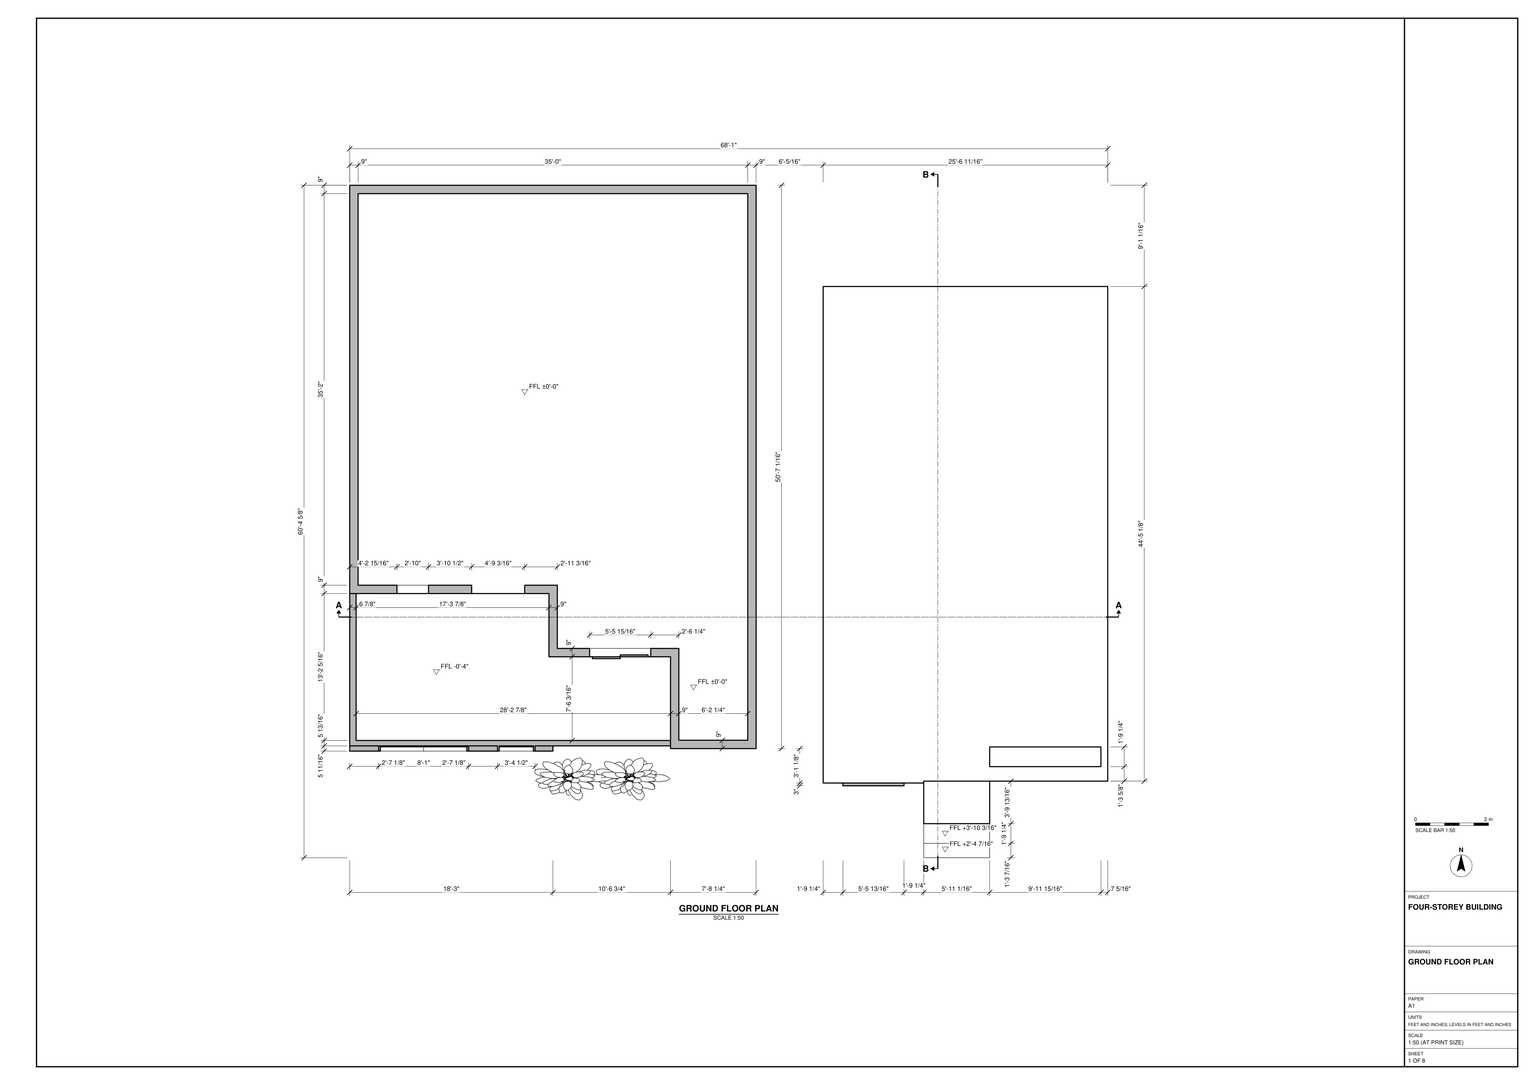
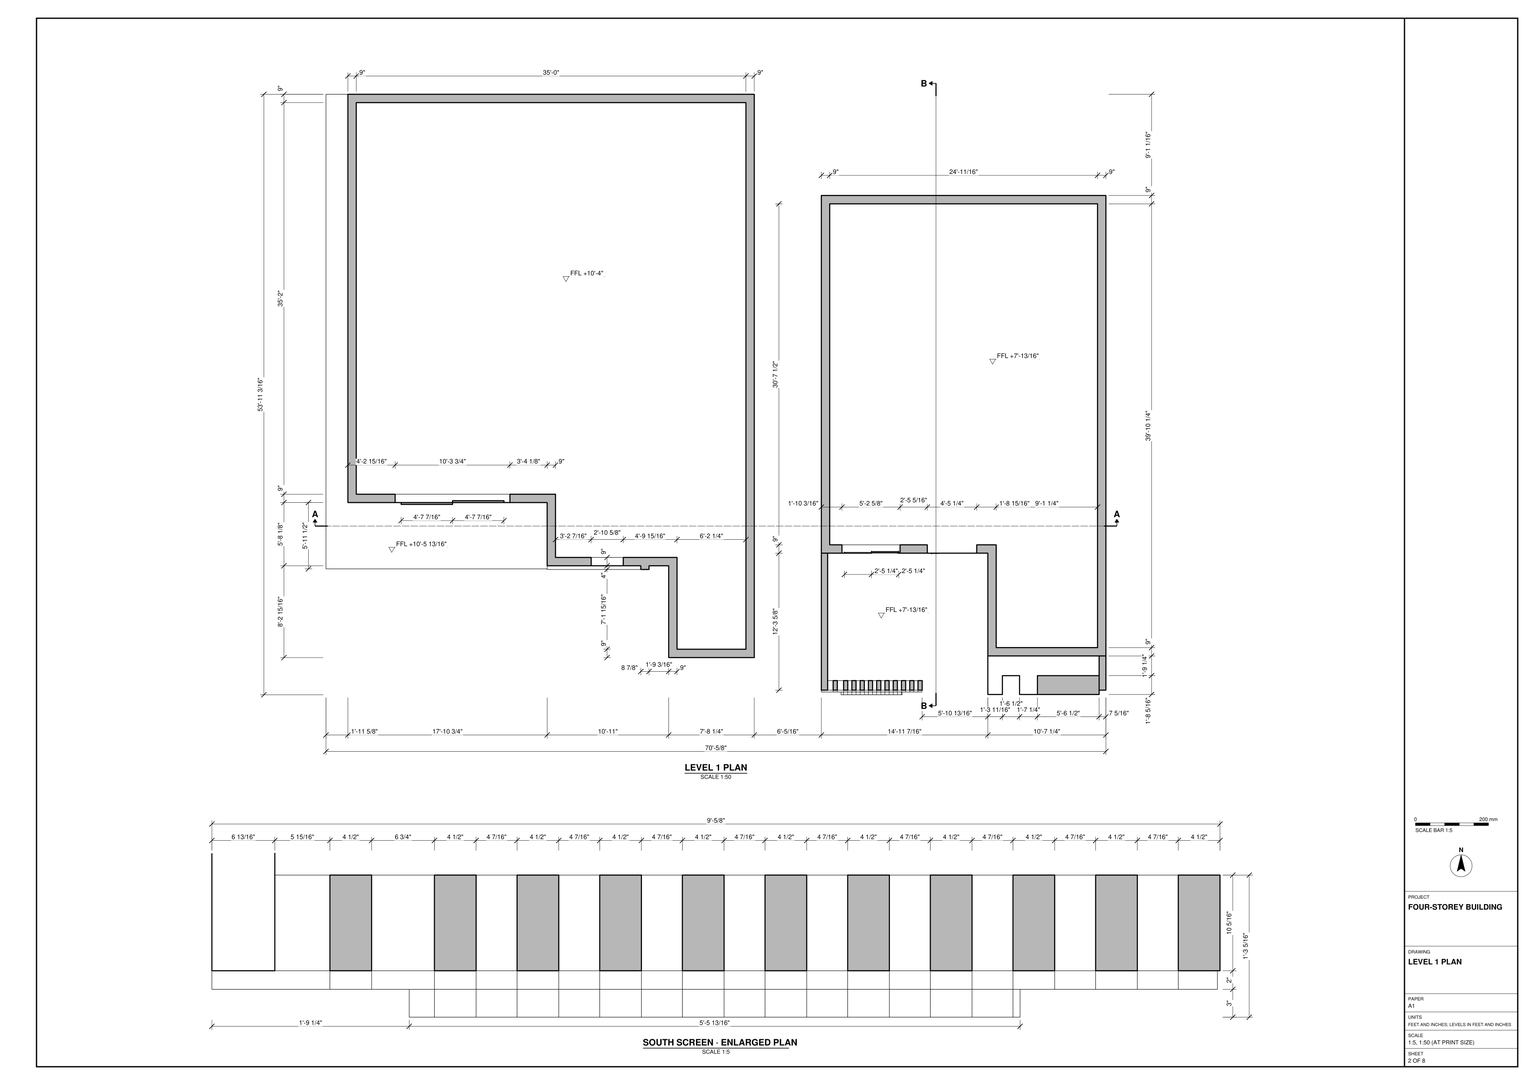
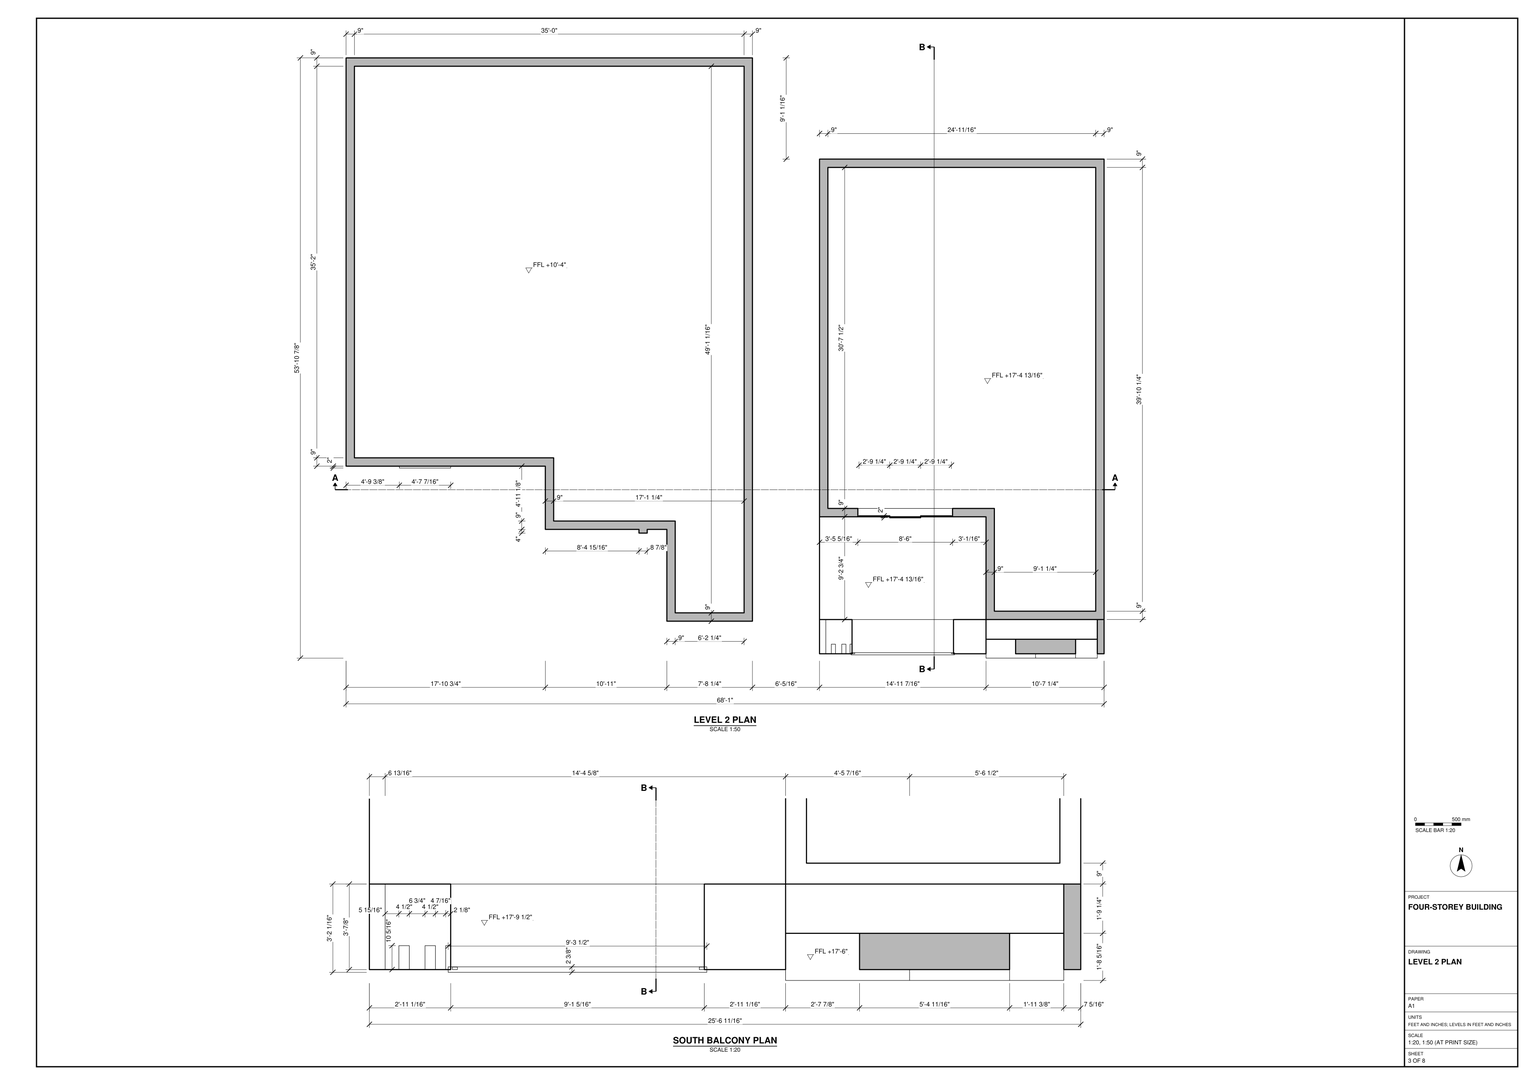
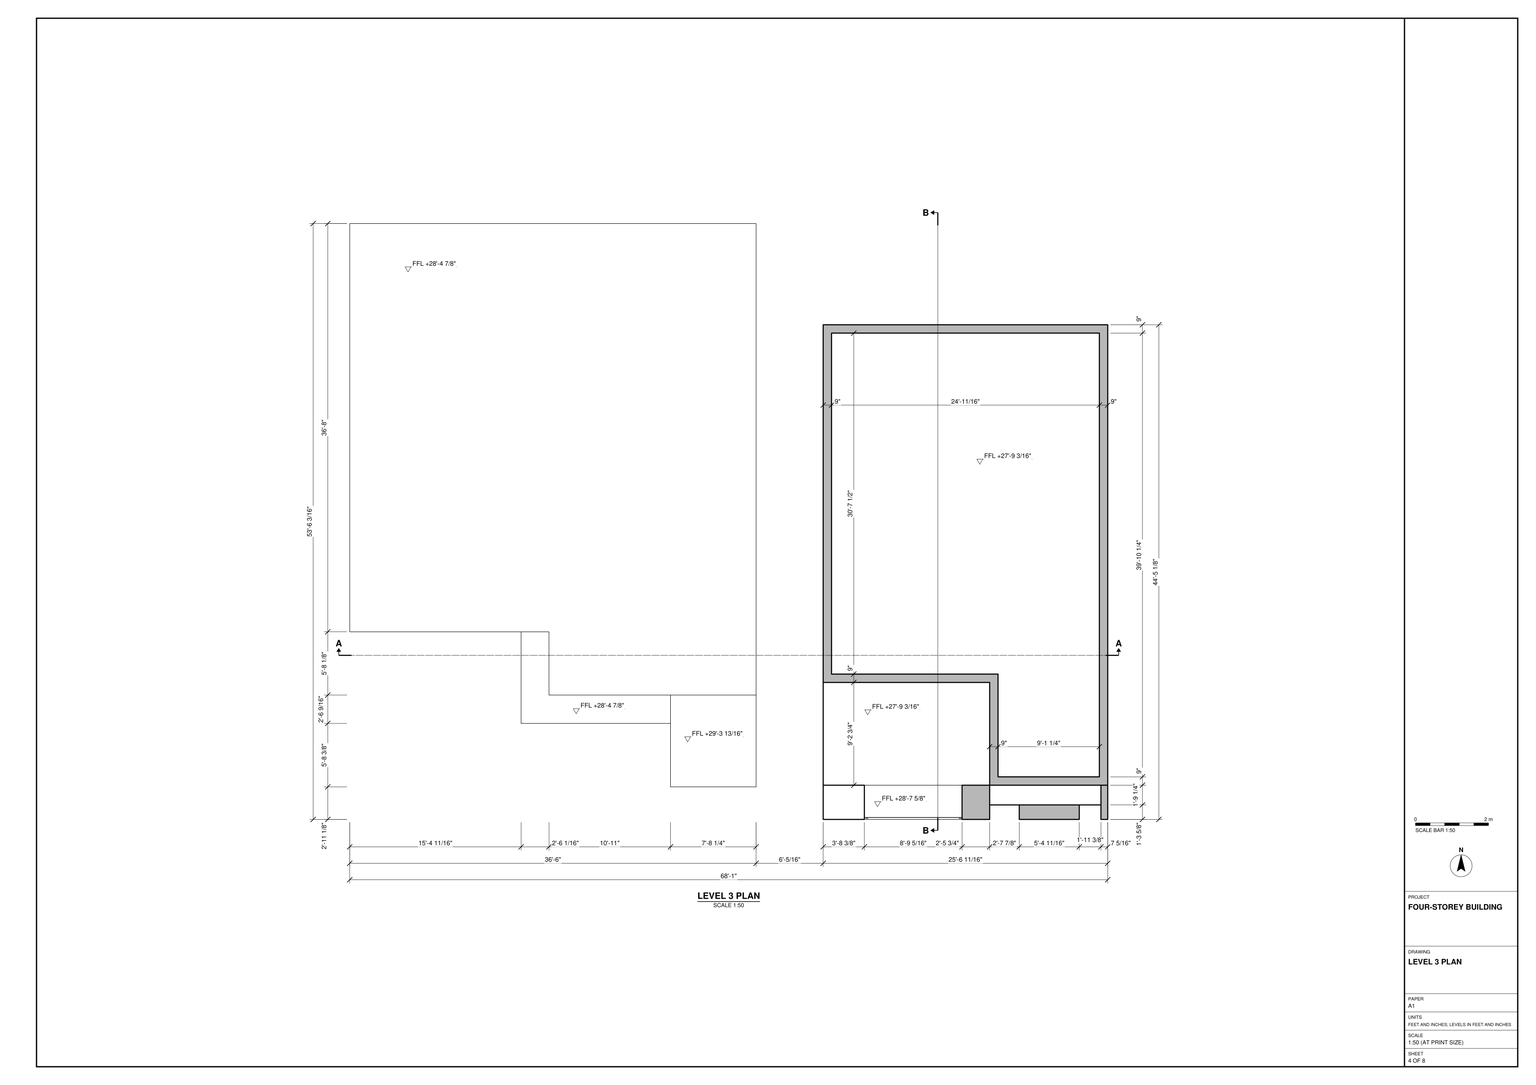
Build the four-storey building in SketchUp from task_files/diagram_01.pdf. Work in feet and inches. The completed model shall measure 70'-5/8" along X, 60'-4 5/8" along Y and 38'-9 3/4" along Z. Use the storey levels ±0'-0", +10'-4", +17'-4 13/16" and +28'-4 7/8" relative to the ground floor. Follow the floor levels marked in each wing rather than extending every slab across both wings.

Place the wider wing to the west and the narrower wing to the east, with the gap and the north–south offset shown in plan. Trace each floor separately to capture the stepped south walls of the west wing and the recessed frontage of the east wing. Model the walls at their drawn thicknesses, including the 9" walls, and place the door and window openings in the corresponding wall segments. Include the floor slabs, entrance steps, roof, and any built-in joinery and main furniture shown. Use the enlarged plans to set out the individual fins of the east wing's south screen and the edges and returns of the balcony above.

Keep walls, slabs, roof elements and individual furniture or joinery pieces in separate groups or components. Use components for repeated parts such as screen fins. Decor and loose items may be any suitable library components. Save one SketchUp model as output_files/four_storey_building_with_offset_wings.skp.

# SketchUp Ruby script. Lengths in inches.
U = 1.inch
M = Sketchup.active_model
def pt(a) = Geom::Point3d.new(a.map { |v| v * U })
def face(e, loops, mat)
  f = e.add_face(loops[0].map { |a| pt(a) })
  loops[1..].each { |l| e.add_face(l.map { |a| pt(a) }).erase! }
  f.material = f.back_material = mat if mat
  f
end
# faces: each face lists its corners as indices into pts; further lists are holes
def faces(e, pts, list, mat = nil) = list.each { |f| face(e, (f[0].is_a?(Array) ? f : [f]).map { |l| l.map { |i| pts[i] } }, mat) }
# xy, xz, yz: faces in a plane at the given z, y or x. An outline is a flat list of corners, or four numbers for a rectangle; further outlines are holes
def ring(l) = l.size == 4 ? [[l[0], l[1]], [l[2], l[1]], [l[2], l[3]], [l[0], l[3]]] : l.each_slice(2).to_a
def flat(e, list, mat, &to3) = list.each { |f| face(e, (f[0].is_a?(Array) ? f : [f]).map { |l| ring(l).map { |u, v| to3.(u, v) } }, mat) }
def xy(e, z, list, mat = nil) = flat(e, list, mat) { |x, y| [x, y, z] }
def xz(e, y, list, mat = nil) = flat(e, list, mat) { |x, z| [x, y, z] }
def yz(e, x, list, mat = nil) = flat(e, list, mat) { |y, z| [x, y, z] }
def lines(e, pts, list) = list.each { |a, b| e.add_line(pt(pts[a]), pt(pts[b])) }
# prism: a flat outline (further loops are holes) pulled along v
def prism(e, loops, v, mat = nil)
  f = face(e, loops, mat); d = Geom::Vector3d.new(v.map { |x| x * U })
  f.pushpull(f.normal.samedirection?(d) ? d.length : -d.length)
end
def box(e, o, s, mat = nil) = prism(e, [[o, [o[0] + s[0], o[1], o[2]], [o[0] + s[0], o[1] + s[1], o[2]], [o[0], o[1] + s[1], o[2]]]], [0, 0, s[2]], mat)
def at(x, y, z, deg = 0) = Geom::Transformation.translation(pt([x, y, z])) * Geom::Transformation.rotation(ORIGIN, Z_AXIS, deg.degrees)
def axes(o, x, y, z) = Geom::Transformation.new([*x, 0, *y, 0, *z, 0, *pt(o).to_a, 1])
def part(name) = M.definitions.add(name)
# library, detail: a bought-in or finely detailed component or shape, given as its bounding box
def library(name, o, s) = part(name).tap { |d| box(d.entities, o, s) }
def detail(e, o, s) = box(e.add_group.entities, o, s)
def put(e, d, t, mat = nil) = e.add_instance(d, t).tap { |i| i.material = mat if mat }
def group(e, t, mat = nil) = e.add_group.tap { |g| g.transformation = t; g.material = mat if mat }.entities
root = M.entities
M.materials.add("Material__1").color = [190, 136, 85]
M.materials.add("Material__2").color = [51, 42, 44]
M.materials.add("Material__3").color = [119, 136, 107]
M.materials.add("[Cladding Weathered]").color = [109, 103, 94]
M.materials.add("[Color C02]").color = [255, 204, 153]
M.materials.add("[Color C07]").color = [153, 76, 0]
M.materials.add("[Color L16]").color = [102, 0, 51]
M.materials.add("[Color M02]").color = [198, 198, 198]
M.materials.add("[Color M03]").color = [170, 170, 170]
M.materials.add("[Color M04]").color = [142, 142, 142]
M.materials.add("[Color M05]").color = [114, 114, 114]
M.materials.add("[Color M06]").color = [86, 86, 86]
M.materials.add("[Color M08]").color = [30, 30, 30]
M.materials.add("[Color M09]").color = [0, 0, 0]
M.materials.add("[Formica Laminate Light]").color = [213, 189, 164]
M.materials.add("[Stone Random Rubble]").color = [91, 91, 91]
M.materials.add("[Stone Vein Gray]").color = [166, 165, 165]
M.materials.add("[Tile Veriegated Stone]").color = [171, 137, 112]
M.materials.add("[Translucent Glass Blue]").color = [7, 17, 153]
M.materials["[Translucent Glass Blue]"].alpha = 0.5
M.materials.add("[Translucent Glass Blue]1").color = [100, 149, 237]
M.materials["[Translucent Glass Blue]1"].alpha = 0.5
M.materials.add("[Translucent Glass Tinted]").color = [8, 201, 241]
M.materials["[Translucent Glass Tinted]"].alpha = 0.48
M.materials.add("[Wood Cherry Original]").color = [152, 86, 42]
c1 = library("\#2",[-119.83,-119.83,113.8],[239.66,239.66,17.4])
c2 = library("\#4",[-204.92,-212.35,-236.71],[424.28,257.5,472.53])
c3 = part("\#3")
put(c3.entities,c2,axes([-0.37,309.72,0],[1.36765,0,0],[0,1.36765,0],[0,0,1.36765]),"Material__3")
c4 = part("Difference\#1")
xy(c4.entities,0,[[345.75,0,345.75,98.9375,324.5625,98.9375,324.5625,94.9375,315.6875,94.9375,315.6875,98.9375,214.75,98.9375,214.75,167.0625,188.59,167.0625,188.59,176.0625,223.75,176.0625,223.75,107.9375,354.75,107.9375,354.75,9,429,9,429,598.0625,9,598.0625,9,176.0625,188.59,176.0625,188.59,167.0625,0,167.0625,0,607.0625,438,607.0625,438,0]])
xy(c4.entities,1.81,[[50.92,167.0625,174.65,176.0625]])
xy(c4.entities,12.375,[[262.1875,98.9375,296.8,107.9375]])
xy(c4.entities,107.98,[[50.92,167.0625,174.65,176.0625]])
xy(c4.entities,124.625,[[262.1875,98.9375,296.8,107.9375]])
xy(c4.entities,138.9,[[0,94.9375,0,167.0625,214.75,167.0625,214.75,98.9375,315.6875,98.9375,315.6875,94.9375]],"[Color M02]")
xy(c4.entities,152.125,[[0,94.9375,324.5625,94.9375,324.5625,98.9375,214.75,98.9375,214.75,167.0625,0,167.0625]],"[Color M08]")
xy(c4.entities,212.875,[[[345.75,0,438,0,438,607.0625,0,607.0625,0,167.0625,214.75,167.0625,214.75,98.9375,345.75,98.9375],[354.75,9,354.75,107.9375,223.75,107.9375,223.75,176.0625,9,176.0625,9,598.0625,429,598.0625,429,9]]])
xz(c4.entities,0,[[345.75,0,438,212.875]])
xz(c4.entities,9,[[354.75,0,429,212.875]])
xz(c4.entities,94.9375,[[315.6875,0,324.5625,0,324.5625,152.125,0,152.125,0,138.9,315.6875,138.9]],"[Color M08]")
xz(c4.entities,98.9375,[[324.5625,0,345.75,0,345.75,212.875,214.75,212.875,214.75,152.125,324.5625,152.125],[[214.75,0,315.6875,138.9],[262.1875,12.375,296.8,124.625]]])
xz(c4.entities,107.9375,[[[223.75,0,354.75,212.875],[262.1875,12.375,296.8,124.625]]])
xz(c4.entities,167.0625,[[[0,0,214.75,138.9],[50.92,1.81,174.65,107.98]],[0,138.9,214.75,152.125],[0,152.125,214.75,212.875]])
xz(c4.entities,176.0625,[[[9,0,223.75,212.875],[50.92,1.81,174.65,107.98]]])
xz(c4.entities,598.0625,[[9,0,429,212.875]])
xz(c4.entities,607.0625,[[0,0,438,212.875]])
yz(c4.entities,0,[[167.0625,0,607.0625,212.875]])
yz(c4.entities,0,[[94.9375,138.9,167.0625,152.125]],"[Color M08]")
yz(c4.entities,9,[[176.0625,0,598.0625,212.875]])
yz(c4.entities,50.92,[[167.0625,1.81,176.0625,107.98]])
yz(c4.entities,174.65,[[167.0625,1.81,176.0625,107.98]])
yz(c4.entities,214.75,[[98.9375,0,167.0625,138.9],[98.9375,152.125,167.0625,212.875]])
yz(c4.entities,223.75,[[107.9375,0,176.0625,212.875]])
yz(c4.entities,262.1875,[[98.9375,12.375,107.9375,124.625]])
yz(c4.entities,296.8,[[98.9375,12.375,107.9375,124.625]])
yz(c4.entities,315.6875,[[94.9375,0,98.9375,138.9]])
yz(c4.entities,324.5625,[[94.9375,0,98.9375,152.125]])
yz(c4.entities,345.75,[[0,0,98.9375,212.875]])
yz(c4.entities,354.75,[[9,0,107.9375,212.875]])
yz(c4.entities,429,[[9,0,598.0625,212.875]])
yz(c4.entities,438,[[0,0,607.0625,212.875]])
c5 = part("Group\#3")
box(c5.entities,[0,-2,0],[55.41,2,93.24])
c6 = library("Slatted screen panel \#1",[0,-1,-56.29],[36.84,1,58.71])
c7 = library("Group\#11",[0,-1,-55.71],[93.48,1,58.6])
c8 = part("Difference\#2")
xy(c8.entities,0,[[345.75,0,345.75,98.9375,214.75,98.9375,214.75,167.0625,188.59,167.0625,188.59,176.0625,223.75,176.0625,223.75,107.9375,354.75,107.9375,354.75,9,429,9,429,598.0625,9,598.0625,9,176.0625,131.41,176.0625,131.41,167.0625,0,167.0625,0,607.0625,438,607.0625,438,0]])
xy(c8.entities,12.41,[[50.92,167.0625,84.9,176.0625]])
xy(c8.entities,42.9375,[[258.5625,98.9375,324.49,107.9375]])
xy(c8.entities,93.0625,[[131.41,167.0625,188.59,176.0625]])
xy(c8.entities,98.98,[[50.92,167.0625,84.9,176.0625]])
xy(c8.entities,109.0625,[[258.5625,98.9375,324.49,107.9375]])
xy(c8.entities,120,[[[345.75,0,438,0,438,607.0625,0,607.0625,0,167.0625,214.75,167.0625,214.75,98.9375,345.75,98.9375],[354.75,9,354.75,107.9375,223.75,107.9375,223.75,176.0625,9,176.0625,9,598.0625,429,598.0625,429,9]]])
xz(c8.entities,0,[[345.75,0,438,120]])
xz(c8.entities,9,[[354.75,0,429,120]])
xz(c8.entities,98.9375,[[[214.75,0,345.75,120],[258.5625,42.9375,324.49,109.0625]]])
xz(c8.entities,98.9375,[[[258.5625,42.9375,324.49,109.0625],[261.47,45.85,321.58,106.15]]],"[Color M09]")
xz(c8.entities,107.9375,[[[223.75,0,354.75,120],[258.5625,42.9375,324.49,109.0625]]])
xz(c8.entities,167.0625,[[[0,0,131.41,0,131.41,93.0625,188.59,93.0625,188.59,0,214.75,0,214.75,120,0,120],[50.92,12.41,84.9,98.98]]])
xz(c8.entities,167.0625,[[[50.92,12.41,84.9,98.98],[53.26,14.76,82.56,96.63]]],"[Color M09]")
xz(c8.entities,167.0625,[[53.26,14.76,82.56,96.63]],"[Translucent Glass Tinted]")
xz(c8.entities,176.0625,[[[9,0,9,120,223.75,120,223.75,0,188.59,0,188.59,93.0625,131.41,93.0625,131.41,0],[50.92,12.41,84.9,98.98]]])
xz(c8.entities,598.0625,[[9,0,429,120]])
xz(c8.entities,607.0625,[[0,0,438,120]])
yz(c8.entities,0,[[167.0625,0,607.0625,120]])
yz(c8.entities,9,[[176.0625,0,598.0625,120]])
yz(c8.entities,50.92,[[167.0625,12.41,176.0625,98.98]])
yz(c8.entities,84.9,[[167.0625,12.41,176.0625,98.98]])
yz(c8.entities,131.41,[[167.0625,0,176.0625,93.0625]])
yz(c8.entities,188.59,[[167.0625,0,176.0625,93.0625]])
yz(c8.entities,214.75,[[98.9375,0,167.0625,120]])
yz(c8.entities,223.75,[[107.9375,0,176.0625,120]])
yz(c8.entities,258.5625,[[98.9375,42.9375,107.9375,109.0625]])
yz(c8.entities,324.49,[[98.9375,42.9375,107.9375,109.0625]])
yz(c8.entities,345.75,[[0,0,98.9375,120]])
yz(c8.entities,354.75,[[9,0,107.9375,120]])
yz(c8.entities,429,[[9,0,598.0625,120]])
yz(c8.entities,438,[[0,0,607.0625,120]])
g1 = group(c8.entities,at(261.47,96.9375,45.85))
g2 = group(g1,at(0,2,0),"[Translucent Glass Tinted]")
box(g2,[0,-2,0],[30.05,2,60.3])
g3 = group(g1,at(30.05,4,0),"[Translucent Glass Tinted]")
box(g3,[0,-2,0],[30.05,2,60.3])
c9 = library("\#1",[-174.07,-174.07,0],[348.14,348.14,140])
c10 = part("Difference\#4")
xy(c10.entities,0,[[179.4375,0,179.4375,110.75,167.47,110.75,167.47,119.75,188.4375,119.75,188.4375,9,297.6875,9,297.6875,487.23,9,487.23,9,119.75,114.1875,119.75,114.1875,110.75,0,110.75,0,496.23,306.6875,496.23,306.6875,0]])
xy(c10.entities,25.61,[[22.2,110.75,84.85,119.75]])
xy(c10.entities,90.42,[[22.2,110.75,84.85,119.75]])
xy(c10.entities,102.6875,[[114.1875,110.75,167.47,119.75]])
xy(c10.entities,120,[[[179.4375,0,306.6875,0,306.6875,496.23,0,496.23,0,110.75,179.4375,110.75],[188.4375,9,188.4375,119.75,9,119.75,9,487.23,297.6875,487.23,297.6875,9]]])
xz(c10.entities,0,[[179.4375,0,306.6875,120]])
xz(c10.entities,9,[[188.4375,0,297.6875,120]])
xz(c10.entities,110.75,[[[0,0,114.1875,0,114.1875,102.6875,167.47,102.6875,167.47,0,179.4375,0,179.4375,120,0,120],[22.2,25.61,84.85,90.42]]])
xz(c10.entities,119.75,[[[9,0,9,120,188.4375,120,188.4375,0,167.47,0,167.47,102.6875,114.1875,102.6875,114.1875,0],[22.2,25.61,84.85,90.42]]])
xz(c10.entities,487.23,[[9,0,297.6875,120]])
xz(c10.entities,496.23,[[0,0,306.6875,120]])
yz(c10.entities,0,[[110.75,0,496.23,120]])
yz(c10.entities,9,[[119.75,0,487.23,120]])
yz(c10.entities,22.2,[[110.75,25.61,119.75,90.42]])
yz(c10.entities,84.85,[[110.75,25.61,119.75,90.42]])
yz(c10.entities,114.1875,[[110.75,0,119.75,102.6875]])
yz(c10.entities,167.47,[[110.75,0,119.75,102.6875]])
yz(c10.entities,179.4375,[[0,0,110.75,120]])
yz(c10.entities,188.4375,[[9,0,119.75,120]])
yz(c10.entities,297.6875,[[9,0,487.23,120]])
yz(c10.entities,306.6875,[[0,0,496.23,120]])
c11 = part("Group\#12")
box(c11.entities,[0,0,0],[306.6875,496.23,4])
c12 = part("Difference")
xy(c12.entities,0,[[[179.4375,0,179.4375,110.75,0,110.75,0,496.23,306.6875,496.23,306.6875,0],[188.4375,9,297.6875,9,297.6875,487.23,9,487.23,9,119.75,188.4375,119.75]]])
xy(c12.entities,25.61,[[41.33,110.75,143.35,119.75]])
xy(c12.entities,90.42,[[41.33,110.75,143.35,119.75]])
xy(c12.entities,120,[[[179.4375,0,306.6875,0,306.6875,496.23,0,496.23,0,110.75,179.4375,110.75],[188.4375,9,188.4375,119.75,9,119.75,9,487.23,297.6875,487.23,297.6875,9]]])
xz(c12.entities,0,[[179.4375,0,306.6875,120]])
xz(c12.entities,9,[[188.4375,0,297.6875,120]])
xz(c12.entities,110.75,[[[0,0,179.4375,120],[41.33,25.61,143.35,90.42]]])
xz(c12.entities,119.75,[[[9,0,188.4375,120],[41.33,25.61,143.35,90.42]]])
xz(c12.entities,487.23,[[9,0,297.6875,120]])
xz(c12.entities,496.23,[[0,0,306.6875,120]])
yz(c12.entities,0,[[110.75,0,496.23,120]])
yz(c12.entities,9,[[119.75,0,487.23,120]])
yz(c12.entities,41.33,[[110.75,25.61,119.75,90.42]])
yz(c12.entities,143.35,[[110.75,25.61,119.75,90.42]])
yz(c12.entities,179.4375,[[0,0,110.75,120]])
yz(c12.entities,188.4375,[[9,0,119.75,120]])
yz(c12.entities,297.6875,[[9,0,487.23,120]])
yz(c12.entities,306.6875,[[0,0,496.23,120]])
c13 = part("Difference\#3")
xy(c13.entities,0,[[179.4375,0,179.4375,110.75,167.47,110.75,167.47,119.75,188.4375,119.75,188.4375,9,297.6875,9,297.6875,487.23,9,487.23,9,119.75,114.1875,119.75,114.1875,110.75,0,110.75,0,496.23,306.6875,496.23,306.6875,0],[114.1875,110.75,167.47,119.75]])
xy(c13.entities,120,[[[179.4375,0,306.6875,0,306.6875,496.23,0,496.23,0,110.75,179.4375,110.75],[188.4375,9,188.4375,119.75,9,119.75,9,487.23,297.6875,487.23,297.6875,9]]])
xz(c13.entities,0,[[179.4375,0,306.6875,120]])
xz(c13.entities,9,[[188.4375,0,297.6875,120]])
xz(c13.entities,110.75,[[0,0,179.4375,120]])
xz(c13.entities,119.75,[[9,0,188.4375,120]])
xz(c13.entities,487.23,[[9,0,297.6875,120]])
xz(c13.entities,496.23,[[0,0,306.6875,120]])
yz(c13.entities,0,[[110.75,0,496.23,120]])
yz(c13.entities,9,[[119.75,0,487.23,120]])
yz(c13.entities,179.4375,[[0,0,110.75,120]])
yz(c13.entities,188.4375,[[9,0,119.75,120]])
yz(c13.entities,297.6875,[[9,0,487.23,120]])
yz(c13.entities,306.6875,[[0,0,496.23,120]])
c14 = part("Group28\#1")
box(c14.entities,[711.27,-0.8125,128.69],[2.16,2.16,33.63])
c15 = part("Group29\#1")
box(c15.entities,[820.61,-0.8125,128.69],[2.17,2.16,33.63])
c16 = part("Group31\#1")
box(c16.entities,[711.27,-0.91,162.32],[111.51,2.36,2.37])
c17 = part("Group32\#1")
box(c17.entities,[712.35,-0.71,132.62],[109.35,1.96,1.97])
c18 = library("Group33\#1",[712.35,0.27,134.59],[109.35,0.01,27.73])
c19 = library("Group\#20",[0,-20.3125,-118.5],[66.48,20.3125,125.22])
xy(root,-4,[[30.5,126.31,369.375,126.31,369.375,216.52,238.375,216.52,238.375,284.65,30.5,284.65]])
xy(root,3.92,[[[533.92,80.48,533.92,615.59,840.61,615.59,840.61,82.48,642.3,82.48,642.3,80.48],[713.36,98.11,833.29,119.36]]])
xy(root,28.42,[[642.3,0,713.36,15.42]])
xy(root,46.17,[[642.3,15.42,713.36,36.67]])
xy(root,64.17,[[642.3,36.67,713.36,56.48]])
xy(root,73.4,[[713.36,77.79,840.61,82.48]])
xy(root,84.8,[[642.3,56.48,713.36,82.48],[766.81,77.79,840.61,77.79,840.61,615.59,533.92,615.59,533.92,80.48,642.3,80.48,642.3,82.48,713.36,82.48,713.36,119.36,833.29,119.36,833.29,98.11,766.81,98.11],[713.36,77.79,766.81,98.11],[713.36,98.11,833.29,119.36]])
xy(root,84.86,[[833.29,82.48,840.61,119.36]])
xy(root,103.375,[[729.04,77.79,747.54,98.11]])
xy(root,114.97,[[0,213.18,0,724.65,23.625,724.65,23.625,284.65,238.375,284.65,238.375,213.18]])
xy(root,125.81,[[0,213.18,238.375,213.18,238.375,284.65,23.625,284.65,23.625,724.65,0,724.65]],"[Color M02]")
xy(root,143.25,[[533.92,80.48,546.64,82.48],[546.64,80.48,551.14,82.48],[551.14,80.48,557.91,82.48],[557.91,80.48,562.4,82.48],[562.4,80.48,566.8125,82.48],
  [566.8125,80.48,571.31,82.48],[571.31,80.48,575.72,82.48],[575.72,80.48,580.22,82.48],[580.22,80.48,584.63,82.48],[584.63,80.48,589.125,82.48],
  [589.125,80.48,593.54,82.48],[593.54,80.48,598.03,82.48],[598.03,80.48,602.45,82.48],[602.45,80.48,606.94,82.48],[606.94,80.48,611.36,82.48],
  [611.36,80.48,615.85,82.48],[615.85,80.48,620.26,82.48],[620.26,80.48,624.76,82.48],[624.76,80.48,629.17,82.48],[629.17,80.48,633.67,82.48],
  [633.67,80.48,638.08,82.48],[638.08,80.48,642.3,82.48],[546.64,82.48,551.14,92.79],[557.91,82.48,562.4,92.79],[566.8125,82.48,571.31,92.79],
  [575.72,82.48,580.22,92.79],[584.63,82.48,589.125,92.79],[593.54,82.48,598.03,92.79],[602.45,82.48,606.94,92.79],[611.36,82.48,615.85,92.79],
  [620.26,82.48,624.76,92.79],[629.17,82.48,633.67,92.79],[638.08,82.48,642.58,92.79]])
xy(root,189.25,[[729.04,77.79,747.54,98.11]])
xy(root,204.8,[[546.64,82.48,551.14,92.79],[557.91,82.48,562.4,92.79],[566.8125,82.48,571.31,92.79],[575.72,82.48,580.22,92.79],[584.63,82.48,589.125,92.79],
  [593.54,82.48,598.03,92.79],[602.45,82.48,606.94,92.79],[611.36,82.48,615.85,92.79],[620.26,82.48,624.76,92.79],[629.17,82.48,633.67,92.79],
  [638.08,82.48,642.58,92.79]])
xy(root,210.01,[[713.36,77.79,766.81,77.79,766.81,82.48,745.24,82.48,745.24,98.11,713.36,98.11],[745.24,82.48,766.81,98.11],[766.81,82.48,809.92,98.11]])
xy(root,235.5625,[[609.64,229.11,642.88,230.11],[576.41,230.11,609.64,231.11],[642.88,230.11,676.11,231.11]],"[Translucent Glass Blue]1")
xy(root,298.06,[[609.64,229.11,642.88,230.11],[576.41,230.11,609.64,231.11],[642.88,230.11,676.11,231.11]],"[Translucent Glass Blue]1")
xy(root,326.3125,[[208.3125,185.96,208.3125,284.65,238.375,284.65,238.375,216.52,369.375,216.52,369.375,185.96]])
xy(root,340.875,[[208.3125,185.96,369.375,185.96,369.375,216.52,238.375,216.52,238.375,284.65,208.3125,284.65]],"[Color M03]")
xy(root,343.61,[[578.3,82.48,683.6,119.36]])
xy(root,434.08,[[745.24,82.48,809.92,98.11]])
xy(root,453.17,[[533.92,82.48,683.6,119.36],[683.6,82.48,713.36,119.36],[713.36,82.48,833.29,98.11],[713.36,98.11,833.29,119.36]])
xy(root,461.72,[[533.92,82.48,840.61,119.36]],"[Color M05]")
xz(root,0,[[642.3,8.99,713.36,28.42]],"[Color M06]")
xz(root,15.42,[[642.3,28.42,713.36,46.17]],"[Color M06]")
xz(root,36.67,[[642.3,46.17,713.36,64.17]],"[Color M06]")
xz(root,56.48,[[642.3,64.17,713.36,84.8]],"[Color M06]")
xz(root,77.79,[[713.36,73.4,840.61,84.8]])
xz(root,77.79,[[[713.36,84.8,766.81,210.01],[729.04,103.375,747.54,189.25]]],"[Color C02]")
xz(root,80.48,[[555.1875,3.92,621.03,84.8],[555.1875,84.8,621.03,121.98]])
xz(root,80.48,[[533.92,3.92,555.1875,84.8],[621.03,3.92,642.3,84.8],[533.92,84.8,555.1875,84.8,555.1875,121.98,621.03,121.98,621.03,84.8,642.3,84.8,642.3,143.25,533.92,143.25]],"[Tile Veriegated Stone]")
xz(root,82.48,[[642.3,3.92,713.36,84.8],[713.36,3.92,840.61,73.4],[546.64,143.25,551.14,204.8],[557.91,143.25,562.4,204.8],[566.8125,143.25,571.31,204.8],
  [575.72,143.25,580.22,204.8],[584.63,143.25,589.125,204.8],[593.54,143.25,598.03,204.8],[602.45,143.25,606.94,204.8],[611.36,143.25,615.85,204.8],
  [620.26,143.25,624.76,204.8],[629.17,143.25,633.67,204.8],[638.08,143.25,642.58,204.8],[[745.24,210.01,809.92,434.08],[749.9,214.68,805.26,429.41]],[578.3,333.17,683.6,343.61]])
xz(root,82.48,[[749.9,214.68,805.26,429.41]],"[Cladding Weathered]")
xz(root,82.48,[[833.29,84.86,840.61,84.86,840.61,461.72,533.92,461.72,533.92,453.17,833.29,453.17]],"[Color M05]")
xz(root,82.48,[[683.6,333.17,713.36,453.17]],"[Stone Vein Gray]")
xz(root,92.79,[[546.64,143.25,551.14,204.8],[557.91,143.25,562.4,204.8],[566.8125,143.25,571.31,204.8],[575.72,143.25,580.22,204.8],[584.63,143.25,589.125,204.8],
  [593.54,143.25,598.03,204.8],[602.45,143.25,606.94,204.8],[611.36,143.25,615.85,204.8],[620.26,143.25,624.76,204.8],[629.17,143.25,633.67,204.8],
  [638.08,143.25,642.58,204.8]])
xz(root,98.11,[[713.36,3.92,833.29,84.8],[766.81,84.8,833.29,203.3],[745.24,210.01,809.92,434.08]])
xz(root,98.11,[[729.04,103.375,747.54,189.25],[713.36,210.01,745.24,210.01,745.24,434.08,809.92,434.08,809.92,210.01,833.29,210.01,833.29,453.17,713.36,453.17]],"[Formica Laminate Light]")
xz(root,119.36,[[713.36,3.92,833.29,84.8],[713.36,84.8,833.29,453.17],[833.29,84.86,833.29,453.17,533.92,453.17,533.92,461.72,840.61,461.72,840.61,84.86],[578.3,333.17,683.6,343.61],[683.6,333.17,713.36,453.17]])
xz(root,185.96,[[208.3125,326.3125,369.375,340.875]],"[Color M03]")
xz(root,213.18,[[0,114.97,238.375,125.81]],"[Color M03]")
xz(root,213.18,[[0,125.81,238.375,158.78]],"[Translucent Glass Blue]")
xz(root,216.52,[[238.375,326.3125,369.375,340.875]])
xz(root,216.52,[[[285.8125,136.375,320.43,248.625],[288.54,139.11,317.69,245.89]]],"[Color M09]")
xz(root,216.52,[[288.54,139.11,317.69,245.89]],"[Translucent Glass Tinted]")
xz(root,229.11,[[609.64,235.5625,642.88,298.06]],"[Translucent Glass Blue]1")
xz(root,229.36,[[652.76,127.97,652.9,127.99,653.04,128.04,653.15,128.13,653.24,128.25,653.3,128.39,653.32,128.53,653.3,128.68,653.24,128.8125,653.15,128.93,653.04,129.02,652.9,129.07,652.76,129.09,652.61,129.07,652.47,129.02,652.36,128.93,652.27,128.8125,652.21,128.68,652.19,128.53,652.21,128.39,652.27,128.25,652.36,128.13,652.47,128.04,652.61,127.99]],"[Color L16]")
xz(root,229.67,[[652.76,127.97,652.61,127.99,652.47,128.04,652.36,128.13,652.27,128.25,652.21,128.39,652.19,128.53,652.21,128.68,652.27,128.8125,652.36,128.93,652.47,129.02,652.61,129.07,652.76,129.09,652.9,129.07,653.04,129.02,653.15,128.93,653.24,128.8125,653.3,128.68,653.32,128.53,653.3,128.39,653.24,128.25,653.15,128.13,653.04,128.04,652.9,127.99]])
xz(root,230.11,[[[575.25,234.41,677.27,299.22],[576.41,235.5625,676.11,298.06]]],"[Color M04]")
xz(root,230.11,[[648.11,84.8,650.82,84.8,650.82,184.78,698.68,184.78,698.68,84.8,701.39,84.8,701.39,187.49,648.11,187.49],[[556.125,110.41,618.77,175.22],[558.72,113,616.18,172.62]]],"[Color M09]")
xz(root,230.11,[[576.41,235.5625,609.64,298.06],[609.64,235.5625,642.88,298.06],[642.88,235.5625,676.11,298.06]],"[Translucent Glass Blue]1")
xz(root,230.11,[[650.82,84.8,698.68,104.79],[650.82,104.79,698.68,124.79],[650.82,124.79,698.68,144.78],[650.82,144.78,698.68,164.78],[650.82,164.78,698.68,184.78]],"[Wood Cherry Original]")
xz(root,231.11,[[576.41,235.5625,609.64,298.06],[642.88,235.5625,676.11,298.06]],"[Translucent Glass Blue]1")
xz(root,281.84,[[161.01,50.38,161.52,50.45,162.01,50.65,162.42,50.96,162.74,51.38,162.9375,51.86,163.01,52.38,162.9375,52.9,162.74,53.38,162.42,53.79,162.01,54.11,161.52,54.31,161.01,54.38,160.49,54.31,160.01,54.11,159.59,53.79,159.27,53.38,159.07,52.9,159.01,52.38,159.07,51.86,159.27,51.38,159.59,50.96,160.01,50.65,160.49,50.45]],"[Color M09]")
xz(root,284.65,[[23.625,114.97,238.375,125.81],[208.3125,326.3125,238.375,340.875]])
xz(root,284.65,[[[158.54,0,208.71,89.56],[161.01,50.38,160.49,50.45,160.01,50.65,159.59,50.96,159.27,51.38,159.07,51.86,159.01,52.38,159.07,52.9,159.27,53.38,159.59,53.79,160.01,54.11,160.49,54.31,161.01,54.38,161.52,54.31,162.01,54.11,162.42,53.79,162.74,53.38,162.9375,52.9,163.01,52.38,162.9375,51.86,162.74,51.38,162.42,50.96,162.01,50.65,161.52,50.45]]],"[Color C07]")
xz(root,284.65,[[155.04,0,158.54,0,158.54,89.56,208.71,89.56,208.71,0,212.21,0,212.21,93.0625,155.04,93.0625],[[74.54,125.81,198.28,231.98],[81,132.28,191.82,225.52]]],"[Color M09]")
xz(root,615.59,[[533.92,3.92,840.61,84.8]])
xz(root,724.65,[[0,114.97,23.625,125.81]])
yz(root,0,[[213.18,114.97,724.65,125.81]],"[Color M03]")
yz(root,0,[[213.18,125.81,407.86,158.78]],"[Translucent Glass Blue]")
yz(root,23.625,[[284.65,114.97,724.65,125.81]])
yz(root,208.3125,[[185.96,326.3125,284.65,340.875]],"[Color M03]")
yz(root,238.375,[[213.18,114.97,284.65,125.81],[216.52,326.3125,284.65,340.875]])
yz(root,369.375,[[185.96,326.3125,216.52,340.875]])
yz(root,533.92,[[80.48,3.92,615.59,84.8],[80.48,84.8,82.48,143.25],[82.48,453.17,119.36,461.72]])
yz(root,533.92,[[119.36,208.8,230.11,329.17],[119.36,333.17,230.11,453.17]],"[Formica Laminate Light]")
yz(root,546.64,[[82.48,143.25,92.79,204.8]])
yz(root,551.14,[[82.48,143.25,92.79,204.8]])
yz(root,557.91,[[82.48,143.25,92.79,204.8]])
yz(root,562.4,[[82.48,143.25,92.79,204.8]])
yz(root,566.8125,[[82.48,143.25,92.79,204.8]])
yz(root,571.31,[[82.48,143.25,92.79,204.8]])
yz(root,575.72,[[82.48,143.25,92.79,204.8]])
yz(root,576.41,[[230.11,235.5625,231.11,298.06]],"[Translucent Glass Blue]1")
yz(root,578.3,[[82.48,333.17,119.36,343.61]])
yz(root,580.22,[[82.48,143.25,92.79,204.8]])
yz(root,584.63,[[82.48,143.25,92.79,204.8]])
yz(root,589.125,[[82.48,143.25,92.79,204.8]])
yz(root,593.54,[[82.48,143.25,92.79,204.8]])
yz(root,598.03,[[82.48,143.25,92.79,204.8]])
yz(root,602.45,[[82.48,143.25,92.79,204.8]])
yz(root,606.94,[[82.48,143.25,92.79,204.8]])
yz(root,609.64,[[229.11,235.5625,230.11,298.06],[230.11,235.5625,231.11,298.06]],"[Translucent Glass Blue]1")
yz(root,611.36,[[82.48,143.25,92.79,204.8]])
yz(root,615.85,[[82.48,143.25,92.79,204.8]])
yz(root,620.26,[[82.48,143.25,92.79,204.8]])
yz(root,624.76,[[82.48,143.25,92.79,204.8]])
yz(root,629.17,[[82.48,143.25,92.79,204.8]])
yz(root,633.67,[[82.48,143.25,92.79,204.8]])
yz(root,638.08,[[82.48,143.25,92.79,204.8]])
yz(root,642.3,[[80.48,3.92,82.48,3.92,80.48,4.05],[82.48,3.92,80.48,4.05,80.48,84.8,82.48,84.8],[80.48,4.05,0,8.99,0,28.42,15.42,28.42,15.42,46.17,36.67,46.17,36.67,64.17,56.48,64.17,56.48,84.8,80.48,84.8],[80.48,84.8,82.48,143.25]])
yz(root,642.58,[[82.48,143.25,92.79,204.8]])
yz(root,642.88,[[229.11,235.5625,230.11,298.06],[230.11,235.5625,231.11,298.06]],"[Translucent Glass Blue]1")
yz(root,676.11,[[230.11,235.5625,231.11,298.06]],"[Translucent Glass Blue]1")
yz(root,683.6,[[82.48,343.61,119.36,453.17]])
yz(root,713.36,[[82.48,3.92,82.48,73.4,77.79,73.4,77.79,84.8,56.48,84.8,56.48,64.17,36.67,64.17,36.67,46.17,15.42,46.17,15.42,28.42,0,28.42,0,8.99],[98.11,3.92,119.36,84.8],[77.79,73.4,82.48,84.8],[82.48,333.17,98.11,453.17],[98.11,333.17,119.36,453.17]])
yz(root,713.36,[[77.79,84.8,77.79,210.01,98.11,210.01,98.11,333.17,119.36,333.17,119.36,84.8]],"[Formica Laminate Light]")
yz(root,729.04,[[77.79,103.375,98.11,189.25]])
yz(root,745.24,[[82.48,210.01,98.11,434.08]])
yz(root,747.54,[[77.79,103.375,98.11,189.25]],"[Formica Laminate Light]")
yz(root,766.81,[[77.79,84.8,98.11,210.01]])
yz(root,809.92,[[82.48,210.01,98.11,434.08]])
yz(root,833.29,[[98.11,3.92,119.36,84.8],[98.11,84.8,119.36,84.86],[82.48,84.86,98.11,453.17],[98.11,84.86,119.36,453.17]])
yz(root,840.61,[[82.48,3.92,615.59,3.92,615.59,84.8,77.79,84.8,77.79,73.4,82.48,73.4],[82.48,84.86,119.36,461.72]])
p = [[642.3,0,8.99],[642.3,80.48,4.05],[642.3,82.48,3.92],[713.36,82.48,3.92],[713.36,0,8.99],[160.01,284.65,50.65],
  [160.49,284.65,50.45],[160.49,281.84,50.45],[160.01,281.84,50.65],[161.01,284.65,50.38],[161.01,281.84,50.38],[161.52,284.65,50.45],
  [161.52,281.84,50.45],[162.01,284.65,50.65],[162.01,281.84,50.65],[159.59,284.65,50.96],[159.59,281.84,50.96],[162.42,284.65,50.96],
  [162.42,281.84,50.96],[159.27,284.65,51.38],[159.27,281.84,51.38],[162.74,284.65,51.38],[162.74,281.84,51.38],[159.07,284.65,51.86],
  [159.07,281.84,51.86],[162.9375,284.65,51.86],[162.9375,281.84,51.86],[159.01,284.65,52.38],[159.01,281.84,52.38],[163.01,284.65,52.38],
  [163.01,281.84,52.38],[159.07,284.65,52.9],[159.07,281.84,52.9],[162.9375,284.65,52.9],[162.9375,281.84,52.9],[159.27,284.65,53.38],
  [159.27,281.84,53.38],[162.74,284.65,53.38],[162.74,281.84,53.38],[159.59,284.65,53.79],[159.59,281.84,53.79],[162.42,284.65,53.79],
  [162.42,281.84,53.79],[160.01,284.65,54.11],[160.01,281.84,54.11],[162.01,284.65,54.11],[162.01,281.84,54.11],[160.49,284.65,54.31],
  [160.49,281.84,54.31],[161.52,284.65,54.31],[161.52,281.84,54.31],[161.01,284.65,54.38],[161.01,281.84,54.38],[652.36,229.67,128.13],
  [652.47,229.67,128.04],[652.47,229.36,128.04],[652.36,229.36,128.13],[652.61,229.67,127.99],[652.61,229.36,127.99],[652.76,229.67,127.97],
  [652.76,229.36,127.97],[652.9,229.67,127.99],[652.9,229.36,127.99],[653.04,229.67,128.04],[653.04,229.36,128.04],[653.15,229.67,128.13],
  [653.15,229.36,128.13],[652.27,229.67,128.25],[652.27,229.36,128.25],[653.24,229.67,128.25],[653.24,229.36,128.25],[652.21,229.67,128.39],
  [652.21,229.36,128.39],[653.3,229.67,128.39],[653.3,229.36,128.39],[652.19,229.67,128.53],[652.19,229.36,128.53],[653.32,229.67,128.53],
  [653.32,229.36,128.53],[652.21,229.67,128.68],[652.21,229.36,128.68],[653.3,229.67,128.68],[653.3,229.36,128.68],[652.27,229.67,128.8125],
  [652.27,229.36,128.8125],[653.24,229.67,128.8125],[653.24,229.36,128.8125],[652.36,229.67,128.93],[652.36,229.36,128.93],[653.15,229.67,128.93],
  [653.15,229.36,128.93],[652.47,229.67,129.02],[652.47,229.36,129.02],[653.04,229.67,129.02],[653.04,229.36,129.02],[652.61,229.67,129.07],
  [652.61,229.36,129.07],[652.9,229.67,129.07],[652.9,229.36,129.07],[652.76,229.67,129.09],[652.76,229.36,129.09],[461.625,117.59,351.8125],
  [369.375,117.59,351.8125],[369.375,216.52,351.8125],[713.36,230.11,84.8],[713.36,202.17,84.8]]
faces(root,p,[[0,1,2,3,4]])
faces(root,p,[[5,6,7,8],[6,9,10,7],[9,11,12,10],[11,13,14,12],[15,5,8,16],[13,17,18,14],[19,15,16,20],[17,21,22,18],
  [23,19,20,24],[21,25,26,22],[27,23,24,28],[25,29,30,26],[31,27,28,32],[29,33,34,30],[35,31,32,36],[33,37,38,34],
  [39,35,36,40],[37,41,42,38],[43,39,40,44],[41,45,46,42],[47,43,44,48],[45,49,50,46],[51,47,48,52],[49,51,52,50]],"[Color C07]")
faces(root,p,[[53,54,55,56],[54,57,58,55],[57,59,60,58],[59,61,62,60],[61,63,64,62],[63,65,66,64],[67,53,56,68],[65,69,70,66],
  [71,67,68,72],[69,73,74,70],[75,71,72,76],[73,77,78,74],[79,75,76,80],[77,81,82,78],[83,79,80,84],[81,85,86,82],
  [87,83,84,88],[85,89,90,86],[91,87,88,92],[89,93,94,90],[95,91,92,96],[93,97,98,94],[99,95,96,100],[97,99,100,98]],"[Color M09]")
lines(root,p,[[101,102],[102,103],[104,105]])
put(root,c1,axes([259.4,86.02,-2.47],[0.12348,0,0],[0,0.07528,0],[0,0,0.11348]),"Material__2")
put(root,c3,axes([264.05,85.43,2.1],[0.03667,0.07188,0],[-0.02643,0.00501,0.11059],[0.11491,-0.02178,0.02543]))
put(root,c1,axes([325.78,86.02,-2.47],[0.12348,0,0],[0,0.07528,0],[0,0,0.11348]),"Material__2")
put(root,c3,axes([330.42,85.43,2.1],[0.03667,0.07188,0],[-0.02643,0.00501,0.11059],[0.11491,-0.02178,0.02543]))
put(root,c4,at(23.625,117.59,124),"[Color M03]")
g4 = group(root,at(238.375,216.52,116.875),"[Color M02]")
xy(g4,0,[[0,-4,109.8125,0]])
xy(g4,7.125,[[0,-4,109.8125,0]])
xz(g4,-4,[[0,0,109.8125,7.125]],"[Color M08]")
xz(g4,0,[[0,0,109.8125,7.125]])
yz(g4,0,[[-4,0,0,7.125]])
yz(g4,109.8125,[[-4,0,0,7.125]])
g5 = group(root,at(81,282.65,132.28))
put(g5,c5,at(0,2,0),"[Translucent Glass Tinted]")
put(g5,c5,at(55.41,4,0),"[Translucent Glass Tinted]")
g6 = group(root,at(23.625,120.52,-4),"[Color M03]")
xy(g6,0,[[159.27,-5.6875,159.27,0,0,0,0,164.125,6.875,164.125,6.875,5.78,345.75,5.78,345.75,0,199.78,0,199.78,-5.6875]])
xy(g6,1.83,[[161.1,-5.6875,197.95,0]],"[Color M09]")
xy(g6,60.54,[[161.1,-5.6875,197.95,0]],"[Color M09]")
xy(g6,62.375,[[159.27,-5.6875,199.78,-5.6875,199.78,0,345.75,0,345.75,5.78,6.875,5.78,6.875,164.125,0,164.125,0,0,159.27,0]])
xz(g6,-5.6875,[[[159.27,0,199.78,62.375],[161.1,1.83,197.95,60.54]]],"[Color M09]")
xz(g6,0,[[0,0,31.15,62.375],[128.125,0,159.27,62.375],[199.78,0,208.375,62.375],[161.1,1.83,197.95,58.125],[33.03,1.89,79.64,57.6],
  [79.64,1.89,126.24,60.49]])
xz(g6,0,[[208.375,0,345.75,62.375]],"[Stone Random Rubble]")
xz(g6,5.78,[[6.875,0,345.75,62.375]])
xz(g6,164.125,[[0,0,6.875,62.375]])
yz(g6,0,[[0,0,164.125,62.375]])
yz(g6,6.875,[[5.78,0,164.125,62.375]])
yz(g6,159.27,[[-5.6875,0,0,62.375]],"[Color M09]")
yz(g6,161.1,[[-5.6875,1.83,0,58.125],[-5.6875,58.125,0,60.54]],"[Color M09]")
yz(g6,197.95,[[-5.6875,1.83,0,58.125],[-5.6875,58.125,0,60.54]],"[Color M09]")
yz(g6,199.78,[[-5.6875,0,0,62.375]],"[Color M09]")
yz(g6,345.75,[[0,0,5.78,62.375]])
put(g6,c6,at(161.1,0,58.125),"[Color M04]")
g7 = group(g6,at(0,0,0))
xy(g7,0,[[0,-5.6875,31.15,0],[128.125,-5.6875,159.27,0],[199.78,-5.6875,218.98,0]])
xy(g7,81.625,[[0,-5.6875,31.15,0],[128.125,-5.6875,159.27,0],[199.78,-5.6875,218.98,0]])
xz(g7,-5.6875,[[0,0,31.15,81.625],[128.125,0,159.27,81.625],[199.78,0,218.98,81.625]],"[Stone Random Rubble]")
xz(g7,0,[[0,0,31.15,81.625],[128.125,0,159.27,81.625],[199.78,0,218.98,81.625]])
yz(g7,0,[[-5.6875,0,0,81.625]])
yz(g7,31.15,[[-5.6875,0,0,81.625]])
yz(g7,128.125,[[-5.6875,0,0,81.625]])
yz(g7,159.27,[[-5.6875,0,0,81.625]])
yz(g7,199.78,[[-5.6875,0,0,81.625]])
yz(g7,218.98,[[-5.6875,0,0,81.625]])
g8 = group(g6,at(31.15,0,0),"[Color M09]")
prism(g8,[[[96.98,0,0],[0,0,0],[0,0,62.375],[96.98,0,62.375]],[[95.09,0,60.49],[48.49,0,60.49],[1.89,0,60.49],[1.89,0,1.89],[48.49,0,1.89],[95.09,0,1.89]]],[0,-5.6875,0])
put(g6,c7,at(33.03,0,57.6),"[Color M04]")
g9 = group(root,at(23.625,117.59,120),"[Color M03]")
prism(g9,[[[0,167.0625,0],[0,607.0625,0],[438,607.0625,0],[438,0,0],[345.75,0,0],[345.75,98.9375,0],[214.75,98.9375,0],[214.75,167.0625,0]]],[0,0,4])
prism(g9,[[[0,167.0625,-124],[0,607.0625,-124],[438,607.0625,-124],[438,0,-124],[345.75,0,-124],[345.75,98.9375,-124],[214.75,98.9375,-124],[214.75,167.0625,-124]]],[0,0,4])
xy(g9,216.875,[[345.75,0,345.75,98.9375,214.75,98.9375,214.75,167.0625,0,167.0625,0,607.0625,438,607.0625,438,0]])
xy(g9,220.875,[[214.75,98.9375,438,98.9375,438,607.0625,0,607.0625,0,167.0625,214.75,167.0625]])
xy(g9,231.8125,[[345.75,0,438,98.9375]])
xz(g9,0,[[345.75,216.875,438,231.8125]])
xz(g9,98.9375,[[214.75,216.875,345.75,220.875],[345.75,220.875,438,231.8125]])
xz(g9,167.0625,[[0,216.875,214.75,220.875]])
xz(g9,607.0625,[[0,216.875,438,220.875]])
yz(g9,0,[[167.0625,216.875,607.0625,220.875]])
yz(g9,214.75,[[98.9375,216.875,167.0625,220.875]])
yz(g9,345.75,[[0,216.875,98.9375,231.8125]])
yz(g9,438,[[0,216.875,607.0625,216.875,607.0625,220.875,98.9375,220.875,98.9375,231.8125,0,231.8125]])
put(root,c8,at(23.625,117.59,0),"[Color M03]")
put(root,c9,axes([259.4,86.02,-2.47],[0.12348,0,0],[0,0.07528,0],[0,0,0.11348]),"Material__1")
put(root,c9,axes([325.78,86.02,-2.47],[0.12348,0,0],[0,0.07528,0],[0,0,0.11348]),"Material__1")
put(root,c10,at(533.92,119.36,84.8),"[Formica Laminate Light]")
put(root,c11,at(533.92,119.36,204.8))
put(root,c12,at(533.92,119.36,208.8),"[Formica Laminate Light]")
put(root,c11,at(533.92,119.36,329.17))
put(root,c13,at(533.92,119.36,333.17),"[Formica Laminate Light]")
g10 = group(root,at(533.92,118.86,204.8),"[Color C02]")
xy(g10,0,[[0,-36.375,179.4375,0.5]])
xy(g10,8.69,[[35.05,-36.375,144.39,0.5]])
xy(g10,93.33,[[35.05,-36.375,144.39,0.5]])
xy(g10,128.375,[[0,-36.375,179.4375,0.5]])
xz(g10,-36.375,[[0,0,6.12,0,6.12,122.26,173.32,122.26,173.32,0,179.4375,0,179.4375,128.375,0,128.375],[6.12,0,35.05,0,35.05,93.33,6.12,122.26],[35.05,0,144.39,8.69],[144.39,0,173.32,0,173.32,122.26,144.39,93.33],[35.05,93.33,144.39,93.33,173.32,122.26,6.12,122.26]])
xz(g10,0.5,[[0,0,0,128.375,179.4375,128.375,179.4375,0,144.39,0,144.39,93.33,35.05,93.33,35.05,0],[35.05,0,144.39,8.69]])
yz(g10,0,[[-36.375,0,0.5,128.375]])
yz(g10,35.05,[[-36.375,8.69,0.5,93.33]])
yz(g10,144.39,[[-36.375,8.69,0.5,93.33]])
yz(g10,179.4375,[[-36.375,0,0.5,128.375]])
put(g10,c14,axes([-675.5,-35.97,-120],[1,0,0],[0,0.5,0],[0,0,1]))
put(g10,c15,axes([-678.39,-35.97,-120],[1,0,0],[0,0.5,0],[0,0,1]))
put(g10,c16,at(-677.31,-36.65,-123.875))
put(g10,c17,at(-677.31,-36.65,-123.875))
put(g10,c18,at(-677.31,-36.65,-123.875))
put(g10,c18,axes([-627.33,-35.54,6.19],[0.94437,0,0],[0,0.91667,0],[0,0,1]))
put(g10,c14,axes([-625.62,-34.92,10.07],[0.94437,0,0],[0,0.45833,0],[0,0,1]))
put(g10,c15,axes([-628.35,-34.92,10.07],[0.94437,0,0],[0,0.45833,0],[0,0,1]))
put(g10,c17,axes([-627.33,-35.54,6.19],[0.94437,0,0],[0,0.91667,0],[0,0,1]))
put(g10,c16,axes([-627.33,-35.54,6.19],[0.94437,0,0],[0,0.91667,0],[0,0,1]))
g11 = group(root,at(533.92,117.86,333.17),"[Cladding Weathered]")
box(g11,[0,-35.375,0],[44.375,36.875,120])
g12 = group(root,at(533.92,82.48,84.8),"[Formica Laminate Light]")
box(g12,[0,0,0],[6.78,147.625,120])
g13 = group(root,at(540.7,82.48,84.8))
box(g13,[0,0,0],[101.87,10.3125,58.45])
g14 = group(root,at(652.76,230.11,127.97),"[Color M09]")
box(g14,[0,-0.4375,0],[7.8125,0.4375,1.125],"[Color M09]")
g15 = group(root,at(558.72,230.11,113),"[Translucent Glass Blue]1")
xy(g15,0,[[0,0,29.27,1]])
xy(g15,59.62,[[0,0,29.27,1]])
xz(g15,0,[[0,0,29.27,59.62]])
yz(g15,0,[[0,0,1,59.62]])
yz(g15,29.27,[[0,0,1,59.62]])
g16 = group(root,at(587.99,231.11,113),"[Translucent Glass Blue]1")
xy(g16,0,[[0,0,29.27,1]])
xy(g16,59.62,[[0,0,29.27,1]])
xz(g16,0,[[0,0,29.27,59.62]])
yz(g16,0,[[0,0,1,59.62]])
yz(g16,29.27,[[0,0,1,59.62]])
put(root,c19,at(766.81,98.11,203.3),"[Color M06]")
put(root,c11,at(533.92,119.36,453.17),"[Formica Laminate Light]")
g17 = group(root,at(555.1875,77.48,3.92),"[Color C02]")
prism(g17,[[[65.84,0,0],[65.84,0,80.875],[65.84,0,118.06],[65.08,0,118.06],[60.66,0,118.06],[56.17,0,118.06],[51.75,0,118.06],[47.26,0,118.06],[42.85,0,118.06],[38.35,0,118.06],[33.9375,0,118.06],[29.44,0,118.06],[25.03,0,118.06],[20.53,0,118.06],[16.12,0,118.06],[11.625,0,118.06],[7.21,0,118.06],[2.72,0,118.06],[0,0,118.06],[0,0,80.875],[0,0,0]]],[0,3,0])
